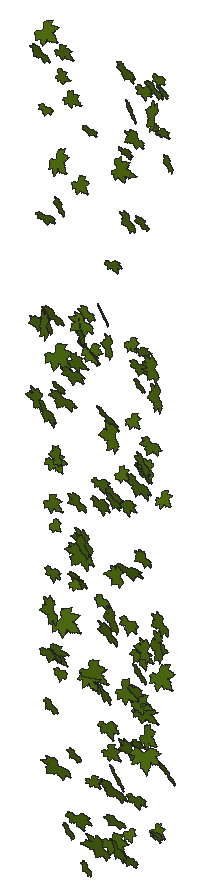
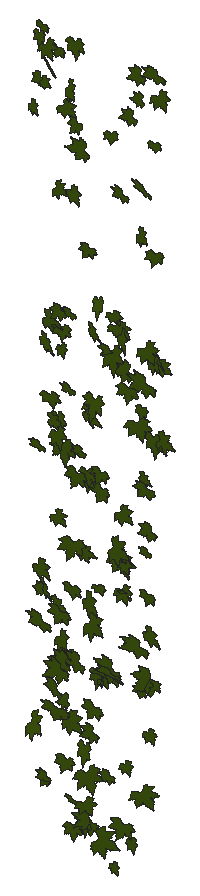
# SketchUp Ruby script. Lengths in inches.
U = 1.inch
M = Sketchup.active_model
def pt(a) = Geom::Point3d.new(a.map { |v| v * U })
def face(e, loops, mat)
  f = e.add_face(loops[0].map { |a| pt(a) })
  loops[1..].each { |l| e.add_face(l.map { |a| pt(a) }).erase! }
  f.material = f.back_material = mat if mat
  f
end
# faces: each face lists its corners as indices into pts; further lists are holes
def faces(e, pts, list, mat = nil) = list.each { |f| face(e, (f[0].is_a?(Array) ? f : [f]).map { |l| l.map { |i| pts[i] } }, mat) }
# xy, xz, yz: faces in a plane at the given z, y or x. An outline is a flat list of corners, or four numbers for a rectangle; further outlines are holes
def ring(l) = l.size == 4 ? [[l[0], l[1]], [l[2], l[1]], [l[2], l[3]], [l[0], l[3]]] : l.each_slice(2).to_a
def flat(e, list, mat, &to3) = list.each { |f| face(e, (f[0].is_a?(Array) ? f : [f]).map { |l| ring(l).map { |u, v| to3.(u, v) } }, mat) }
def xy(e, z, list, mat = nil) = flat(e, list, mat) { |x, y| [x, y, z] }
def xz(e, y, list, mat = nil) = flat(e, list, mat) { |x, z| [x, y, z] }
def yz(e, x, list, mat = nil) = flat(e, list, mat) { |y, z| [x, y, z] }
def lines(e, pts, list) = list.each { |a, b| e.add_line(pt(pts[a]), pt(pts[b])) }
# prism: a flat outline (further loops are holes) pulled along v
def prism(e, loops, v, mat = nil)
  f = face(e, loops, mat); d = Geom::Vector3d.new(v.map { |x| x * U })
  f.pushpull(f.normal.samedirection?(d) ? d.length : -d.length)
end
def box(e, o, s, mat = nil) = prism(e, [[o, [o[0] + s[0], o[1], o[2]], [o[0] + s[0], o[1] + s[1], o[2]], [o[0], o[1] + s[1], o[2]]]], [0, 0, s[2]], mat)
def at(x, y, z, deg = 0) = Geom::Transformation.translation(pt([x, y, z])) * Geom::Transformation.rotation(ORIGIN, Z_AXIS, deg.degrees)
def axes(o, x, y, z) = Geom::Transformation.new([*x, 0, *y, 0, *z, 0, *pt(o).to_a, 1])
def part(name) = M.definitions.add(name)
# library, detail: a bought-in or finely detailed component or shape, given as its bounding box
def library(name, o, s) = part(name).tap { |d| box(d.entities, o, s) }
def detail(e, o, s) = box(e.add_group.entities, o, s)
def put(e, d, t, mat = nil) = e.add_instance(d, t).tap { |i| i.material = mat if mat }
def group(e, t, mat = nil) = e.add_group.tap { |g| g.transformation = t; g.material = mat if mat }.entities
root = M.entities
M.materials.add("[Vegetation Blur 03]").color = [83, 114, 18]
c1 = part("ivy")
xy(c1.entities,0,[[0.782,0,0.786,0,0.787,0.005,0.789,0.009,0.821,0.072,0.875,0.147,1.001,0.272,1.073,0.331,1.137,0.363,1.178,0.379,1.223,0.384,1.272,0.383,1.311,0.374,1.36,0.355,1.399,0.334,1.491,0.285,1.541,0.244,1.583,0.199,1.617,0.15,1.64,0.128,1.662,0.115,1.717,0.105,1.745,0.093,1.784,0.054,1.819,0.057,1.854,0.064,1.882,0.075,1.896,0.074,1.91,0.071,1.937,0.063,1.964,0.053,1.99,0.038,2.016,0.015,2.034,0.002,2.04,0,2.038,0.003,2.036,0.007,2.033,0.038,2.036,0.068,2.045,0.1,2.055,0.116,2.064,0.123,2.077,0.129,2.088,0.129,2.106,0.132,2.118,0.13,2.179,0.132,2.207,0.133,2.225,0.133,2.242,0.138,2.22,0.162,2.207,0.186,2.206,0.213,2.212,0.236,2.228,0.262,2.247,0.274,2.298,0.283,2.355,0.294,2.37,0.296,2.376,0.295,2.377,0.3,2.377,0.303,2.385,0.329,2.411,0.37,2.426,0.392,2.449,0.407,2.511,0.426,2.561,0.444,2.619,0.466,2.589,0.469,2.561,0.476,2.501,0.5,2.449,0.516,2.424,0.523,2.401,0.535,2.377,0.556,2.372,0.568,2.36,0.575,2.268,0.586,2.225,0.592,2.207,0.599,2.194,0.61,2.143,0.65,2.13,0.664,2.122,0.682,2.123,0.7,2.13,0.719,2.148,0.75,2.17,0.781,2.195,0.807,2.221,0.828,2.284,0.874,2.291,0.88,2.288,0.887,2.276,0.9,2.267,0.916,2.265,0.933,2.273,0.967,2.292,1.002,2.313,1.03,2.334,1.054,2.348,1.067,2.358,1.074,2.363,1.076,2.362,1.081,2.35,1.094,2.347,1.11,2.35,1.143,2.359,1.18,2.385,1.254,2.415,1.324,2.448,1.393,2.45,1.4,2.446,1.398,2.44,1.394,2.427,1.383,2.402,1.36,2.376,1.339,2.345,1.324,2.305,1.309,2.282,1.303,2.273,1.306,2.245,1.294,2.212,1.287,2.187,1.291,2.163,1.301,2.142,1.316,2.134,1.327,2.124,1.325,2.09,1.292,2.053,1.259,2.014,1.234,1.973,1.215,1.954,1.21,1.931,1.208,1.909,1.212,1.893,1.22,1.879,1.233,1.872,1.248,1.867,1.281,1.864,1.319,1.821,1.258,1.773,1.197,1.726,1.141,1.698,1.121,1.679,1.116,1.666,1.117,1.647,1.122,1.632,1.129,1.62,1.141,1.617,1.154,1.617,1.219,1.621,1.254,1.623,1.268,1.623,1.281,1.618,1.314,1.606,1.346,1.603,1.375,1.607,1.403,1.603,1.467,1.599,1.499,1.605,1.525,1.614,1.552,1.629,1.577,1.635,1.589,1.629,1.587,1.618,1.582,1.596,1.566,1.581,1.556,1.568,1.552,1.557,1.55,1.545,1.553,1.531,1.562,1.522,1.572,1.504,1.591,1.486,1.611,1.474,1.631,1.457,1.666,1.455,1.684,1.457,1.698,1.452,1.715,1.444,1.728,1.424,1.754,1.419,1.772,1.423,1.786,1.434,1.819,1.444,1.848,1.446,1.855,1.44,1.861,1.43,1.867,1.386,1.904,1.349,1.948,1.326,1.973,1.31,1.995,1.288,2.048,1.284,2.153,1.287,2.254,1.284,2.255,1.282,2.253,1.278,2.247,1.274,2.237,1.266,2.216,1.226,2.125,1.208,2.076,1.184,2.033,1.155,1.984,1.135,1.942,1.111,1.899,1.083,1.861,1.053,1.85,1.059,1.83,1.061,1.809,1.056,1.79,1.049,1.767,1.04,1.749,1.018,1.733,0.994,1.726,0.942,1.734,0.95,1.6875,0.944,1.645,0.932,1.608,0.911,1.585,0.881,1.58,0.854,1.582,0.828,1.588,0.785,1.618,0.773,1.625,0.775,1.614,0.779,1.598,0.796,1.502,0.818,1.402,0.861,1.283,0.882,1.224,0.894,1.174,0.892,1.148,0.886,1.123,0.881,1.107,0.872,1.099,0.849,1.094,0.818,1.092,0.789,1.098,0.762,1.107,0.753,1.113,0.721,1.139,0.698,1.163,0.678,1.194,0.665,1.224,0.628,1.28,0.612,1.312,0.606,1.327,0.606,1.314,0.599,1.282,0.594,1.267,0.581,1.256,0.544,1.245,0.512,1.244,0.473,1.249,0.444,1.256,0.382,1.288,0.339,1.306,0.324,1.316,0.317,1.324,0.309,1.326,0.27,1.314,0.227,1.313,0.185,1.3125,0.152,1.317,0.122,1.328,0.092,1.345,0.073,1.353,0.079,1.338,0.092,1.308,0.117,1.249,0.13,1.215,0.139,1.164,0.147,1.148,0.157,1.136,0.163,1.122,0.174,1.086,0.177,1.067,0.182,1.054,0.186,1.043,0.191,1.038,0.211,1.028,0.237,1.005,0.25,0.974,0.253,0.96,0.25,0.944,0.242,0.914,0.243,0.906,0.249,0.902,0.26,0.894,0.289,0.88,0.307,0.873,0.322,0.862,0.364,0.799,0.403,0.738,0.431,0.709,0.439,0.691,0.441,0.678,0.4375,0.66,0.428,0.645,0.394,0.623,0.303,0.594,0.255,0.581,0.214,0.577,0.179,0.573,0.173,0.568,0.175,0.561,0.167,0.55,0.141,0.523,0.113,0.503,0.077,0.49,0.045,0.486,0.026,0.485,0.019,0.486,0.011,0.483,0,0.471,0.014,0.467,0.044,0.455,0.058,0.447,0.07,0.438,0.097,0.411,0.125,0.394,0.158,0.377,0.174,0.366,0.182,0.359,0.185,0.361,0.242,0.331,0.253,0.316,0.258,0.303,0.262,0.283,0.274,0.278,0.308,0.274,0.341,0.252,0.366,0.226,0.366,0.222,0.37,0.22,0.38,0.221,0.395,0.221,0.425,0.216,0.45,0.207,0.465,0.192,0.473,0.178,0.484,0.15,0.489,0.116,0.483,0.089,0.468,0.058,0.45,0.035,0.435,0.018,0.429,0.011,0.434,0.012,0.438,0.014,0.469,0.019,0.542,0.016,0.581,0.015,0.612,0.027,0.68,0.055,0.696,0.057,0.712,0.052,0.73,0.045,0.741,0.036,0.766,0.014]])
put(root,c1,axes([11.16,173.7,30.11],[0.07342,0.0201,-0.45241],[-0.55143,0.12193,-0.05876],[-0.05747,-1.14418,-0.01421]),"[Vegetation Blur 03]")
put(root,c1,axes([11,173.7,33.93],[0.13601,0.05917,-0.30855],[-0.37908,0.03752,-0.11017],[-0.00748,-0.82593,-0.02711]),"[Vegetation Blur 03]")
put(root,c1,axes([10.83,173.7,48.26],[0.33145,0.05992,-0.29685],[-0.36343,0.14447,-0.2657],[-0.03257,-1.00226,-0.05605]),"[Vegetation Blur 03]")
put(root,c1,axes([11.58,173.7,34.26],[0.12192,-0.00071,-0.41999],[-0.49465,0.29998,-0.09572],[-0.14193,-1.04612,-0.02717]),"[Vegetation Blur 03]")
put(root,c1,axes([11.62,173.7,34.28],[0.14174,-0.20689,-0.42841],[-0.51411,0.25268,-0.13249],[-0.14609,-1.08996,0.0506]),"[Vegetation Blur 03]")
put(root,c1,axes([10.85,173.7,39.43],[0.38883,0.03177,-0.00541],[-0.00902,0.12865,-0.31342],[0.01417,-0.78985,-0.05127]),"[Vegetation Blur 03]")
put(root,c1,axes([11.09,173.7,45.22],[0.29737,0.00668,-0.03254],[-0.03987,-0.00069,-0.24271],[0.00326,-0.6174,-0.00008]),"[Vegetation Blur 03]")
put(root,c1,axes([10.63,173.7,48.53],[0.22945,0.18892,0.3925],[0.48869,-0.02142,-0.18866],[0.02999,-1.09631,0.07132]),"[Vegetation Blur 03]")
put(root,c1,axes([11.57,173.7,34.72],[0.32489,0.11128,-0.34401],[-0.42351,0.17483,-0.25752],[-0.03505,-1.08109,-0.07706]),"[Vegetation Blur 03]")
put(root,c1,axes([11.04,173.7,29.73],[0.57169,-0.21875,-0.18427],[-0.21197,0.1873,-0.473],[-0.13171,-1.2509,-0.0386]),"[Vegetation Blur 03]")
put(root,c1,axes([11.55,173.7,14.08],[0.26898,-0.00531,-0.22272],[-0.27011,0.10743,-0.21769],[-0.03898,-0.78115,-0.02842]),"[Vegetation Blur 03]")
put(root,c1,axes([11.86,173.7,19.51],[0.26861,-0.16753,-0.42435],[-0.51691,0.14174,-0.22674],[-0.09889,-1.19591,0.03257]),"[Vegetation Blur 03]")
put(root,c1,axes([11.67,173.7,11.125],[0.44397,0.1395,-0.34863],[-0.43136,0.05055,-0.3627],[0.03168,-1.26682,-0.05286]),"[Vegetation Blur 03]")
put(root,c1,axes([11.64,173.7,16.72],[0.30297,0.01543,-0.16149],[-0.19571,0.1367,-0.2425],[-0.03016,-0.73198,-0.04869]),"[Vegetation Blur 03]")
put(root,c1,axes([12.27,173.7,40.52],[0.10541,0.02404,-0.33372],[-0.3979,0.2077,-0.08136],[-0.09494,-0.84377,-0.02954]),"[Vegetation Blur 03]")
put(root,c1,axes([11.22,173.7,24.11],[0.22933,0.01454,0.32661],[0.40022,0.004,-0.18721],[0.0052,-0.94915,0.00421]),"[Vegetation Blur 03]")
put(root,c1,axes([11.4,173.7,21.01],[0.4011,-0.07198,0.04538],[0.05521,-0.01426,-0.32859],[-0.0356,-0.83315,0.0017]),"[Vegetation Blur 03]")
put(root,c1,axes([10.88,173.7,16.34],[0.50593,-0.03643,0.3437],[0.41936,0.17969,-0.40818],[0.0424,-1.34262,-0.06395]),"[Vegetation Blur 03]")
put(root,c1,axes([12.28,173.7,27.52],[0.12968,-0.11784,-0.31424],[-0.38451,0.09135,-0.11108],[-0.06065,-0.83104,0.03235]),"[Vegetation Blur 03]")
put(root,c1,axes([11.58,173.7,23.08],[0.14273,0.06127,0.20808],[0.25666,-0.04237,-0.11531],[-0.00355,-0.59977,0.0294]),"[Vegetation Blur 03]")
put(root,c1,axes([11.28,173.7,26.49],[0.3729,0.07352,0.23123],[0.28448,-0.01242,-0.30497],[0.02479,-0.96364,0.02157]),"[Vegetation Blur 03]")
put(root,c1,axes([11.84,173.7,30.48],[0.49872,0.09657,-0.2358],[-0.29251,0.12066,-0.4043],[0.0109,-1.17989,-0.06065]),"[Vegetation Blur 03]")
put(root,c1,axes([11.83,173.7,30.86],[0.33145,-0.08577,-0.02014],[-0.01771,0.11215,-0.26935],[-0.04508,-0.6747,-0.04221]),"[Vegetation Blur 03]")
put(root,c1,axes([11.1875,173.7,31.82],[0.38163,0.10723,0.44815],[0.5511,-0.01709,-0.31195],[0.0229,-1.37595,0.0388]),"[Vegetation Blur 03]")
put(root,c1,axes([11.51,173.7,42.07],[0.21319,0.1755,0.40106],[0.49372,-0.23014,-0.15897],[-0.07069,-1.078,0.09923]),"[Vegetation Blur 03]")
put(root,c1,axes([11.95,173.7,15.84],[0.32221,-0.0387,0.02273],[0.02664,-0.04287,-0.26295],[-0.0205,-0.66413,0.01565]),"[Vegetation Blur 03]")
put(root,c1,axes([12.03,173.7,46.77],[0.07701,-0.01607,0.28736],[0.35217,-0.0014,-0.06288],[-0.00233,-0.74167,-0.00611]),"[Vegetation Blur 03]")
put(root,c1,axes([11.58,173.7,17.75],[0.25598,0.2014,0.48378],[0.59803,0.04143,-0.21349],[0.05748,-1.32803,0.06671]),"[Vegetation Blur 03]")
put(root,c1,axes([11.89,173.7,48.13],[0.23882,-0.04134,0.29544],[0.36225,0.06442,-0.19363],[0.01513,-0.89011,-0.02773]),"[Vegetation Blur 03]")
put(root,c1,axes([12.58,173.7,7.89],[0.29522,-0.08617,-0.18688],[-0.21829,0.16177,-0.24143],[-0.08083,-0.75161,-0.03054]),"[Vegetation Blur 03]")
put(root,c1,axes([12.34,173.7,31.86],[0.50551,0.02715,-0.04471],[-0.05585,0.1053,-0.41049],[0.00753,-1.04102,-0.04269]),"[Vegetation Blur 03]")
put(root,c1,axes([12.92,173.7,11.91],[0.2455,0.02361,-0.20397],[-0.24867,0.10235,-0.19749],[-0.02754,-0.71362,-0.03507]),"[Vegetation Blur 03]")
put(root,c1,axes([12.96,173.7,22.6],[0.23892,0.03876,-0.2007],[-0.24369,0.14566,-0.1888],[-0.038,-0.69034,-0.0511]),"[Vegetation Blur 03]")
put(root,c1,axes([13.23,173.7,25.42],[0.22065,0.07279,-0.34055],[-0.41864,0.06201,-0.17859],[-0.01021,-0.96933,-0.037]),"[Vegetation Blur 03]")
put(root,c1,axes([12.4,173.7,45.74],[0.16739,0.00231,0.3142],[0.38437,0.04772,-0.13645],[0.02172,-0.86254,-0.00671]),"[Vegetation Blur 03]")
put(root,c1,axes([12.97,173.7,21.24],[0.33471,0.047,-0.24757],[-0.30145,0.17573,-0.26622],[-0.0408,-0.91277,-0.064]),"[Vegetation Blur 03]")
put(root,c1,axes([12.74,173.7,20.37],[0.12441,0.10653,0.22366],[0.27873,-0.02631,-0.1013],[0.00957,-0.61876,0.04281]),"[Vegetation Blur 03]")
put(root,c1,axes([13.86,173.7,23.6],[0.10808,0.0782,-0.51354],[-0.62715,0.14615,-0.08441],[-0.06373,-1.30565,-0.04021]),"[Vegetation Blur 03]")
put(root,c1,axes([12.96,173.7,22.875],[0.56655,-0.0115,-0.27779],[-0.34007,0.04247,-0.46224],[-0.01542,-1.35941,-0.01209]),"[Vegetation Blur 03]")
put(root,c1,axes([13.29,173.7,34.89],[0.41729,-0.27977,-0.39423],[-0.44817,0.37379,-0.3577],[-0.22574,-1.25924,-0.01859]),"[Vegetation Blur 03]")
put(root,c1,axes([12.51,173.7,8.41],[0.53014,0.02962,0.10212],[0.12282,0.12551,-0.4304],[0.02794,-1.11386,-0.04578]),"[Vegetation Blur 03]")
put(root,c1,axes([13.65,173.7,23.35],[0.21226,-0.08156,-0.39258],[-0.47103,0.20087,-0.17619],[-0.10528,-1.06312,-0.00317]),"[Vegetation Blur 03]")
put(root,c1,axes([12.71,173.7,31.98],[0.16066,-0.07376,0.37357],[0.45903,0.04715,-0.13002],[0.00982,-0.99714,-0.03378]),"[Vegetation Blur 03]")
put(root,c1,axes([13.39,173.7,35.1],[0.38856,-0.00058,-0.29483],[-0.35992,-0.09405,-0.31593],[0.03091,-1.0877,0.02748]),"[Vegetation Blur 03]")
put(root,c1,axes([12.87,173.7,41.5],[0.24024,0.06291,0.29442],[0.3619,-0.06648,-0.19446],[-0.01006,-0.88941,0.03536]),"[Vegetation Blur 03]")
put(root,c1,axes([13.41,173.7,33.74],[0.55985,-0.09656,-0.30764],[-0.35518,0.35678,-0.44814],[-0.13469,-1.34226,-0.09699]),"[Vegetation Blur 03]")
put(root,c1,axes([13.73,173.7,6.25],[0.22842,-0.06235,-0.19773],[-0.23665,0.11144,-0.18763],[-0.06007,-0.67607,-0.01269]),"[Vegetation Blur 03]")
put(root,c1,axes([13.64,173.7,35.52],[0.31144,-0.00755,-0.1936],[-0.23722,0.00118,-0.25419],[-0.00327,-0.80561,0.00144]),"[Vegetation Blur 03]")
put(root,c1,axes([13.61,173.7,44.96],[0.30877,0.02964,-0.06253],[-0.07793,0.09874,-0.24894],[0.00225,-0.64717,-0.04084]),"[Vegetation Blur 03]")
put(root,c1,axes([14.74,173.7,7.86],[0.10967,0.16764,-0.53959],[-0.66571,-0.0227,-0.09123],[0.02429,-1.37893,-0.0641]),"[Vegetation Blur 03]")
put(root,c1,axes([13.22,173.7,15.87],[0.43423,0.11965,0.28912],[0.35873,-0.10053,-0.35232],[0.01383,-1.14881,0.06094]),"[Vegetation Blur 03]")
put(root,c1,axes([13.45,173.7,32.98],[0.34318,0.09184,0.26358],[0.326,-0.10859,-0.27677],[-0.00403,-0.96364,0.05631]),"[Vegetation Blur 03]")
put(root,c1,axes([13.7,173.7,10.47],[0.24944,0.02336,0.19362],[0.23616,0.05082,-0.20362],[0.02524,-0.70655,-0.00824]),"[Vegetation Blur 03]")
put(root,c1,axes([14.39,173.7,15.9],[0.17883,0.01791,-0.19414],[-0.23754,0.05276,-0.14498],[-0.01529,-0.61012,-0.01823]),"[Vegetation Blur 03]")
put(root,c1,axes([13.29,173.7,15.91],[0.34678,0.03788,0.46084],[0.56412,0.05104,-0.28341],[0.03077,-1.36263,0.00219]),"[Vegetation Blur 03]")
put(root,c1,axes([15.08,173.7,19.15],[0.17288,0.13727,-0.46997],[-0.57483,0.20036,-0.13164],[-0.0749,-1.22089,-0.07445]),"[Vegetation Blur 03]")
put(root,c1,axes([14.09,173.7,26.55],[0.40772,-0.01716,0.08723],[0.10718,0.04684,-0.33224],[-0.00228,-0.8661,-0.01969]),"[Vegetation Blur 03]")
put(root,c1,axes([14.53,173.7,20.62],[0.28445,-0.01133,-0.1134],[-0.139,-0.04223,-0.23156],[0.00407,-0.65007,0.01702]),"[Vegetation Blur 03]")
put(root,c1,axes([14.47,173.7,35.88],[0.40706,-0.21039,-0.21028],[-0.21941,0.3311,-0.33502],[-0.1694,-0.93442,-0.07136]),"[Vegetation Blur 03]")
put(root,c1,axes([14.06,173.7,25.625],[0.48848,-0.12647,0.08295],[0.10536,0.05262,-0.40062],[-0.05484,-1.02537,-0.03079]),"[Vegetation Blur 03]")
put(root,c1,axes([14.47,173.7,15.94],[0.464,-0.18688,-0.09777],[-0.10719,0.14954,-0.38378],[-0.10541,-0.97473,-0.04013]),"[Vegetation Blur 03]")
put(root,c1,axes([15.33,173.7,34.38],[0.12813,-0.15006,-0.36786],[-0.44192,0.20151,-0.11546],[-0.11482,-0.94298,0.03387]),"[Vegetation Blur 03]")
put(root,c1,axes([14.77,173.7,11.03],[0.53027,0.09687,-0.32245],[-0.39653,0.24084,-0.42296],[-0.03295,-1.33931,-0.09938]),"[Vegetation Blur 03]")
put(root,c1,axes([14.39,173.7,30.54],[0.61753,-0.18671,-0.12394],[-0.12621,0.33022,-0.49708],[-0.12397,-1.26626,-0.11135]),"[Vegetation Blur 03]")
put(root,c1,axes([15.35,173.7,20.17],[0.24952,-0.09563,-0.45788],[-0.54485,0.27669,-0.20686],[-0.14163,-1.23287,-0.01091]),"[Vegetation Blur 03]")
put(root,c1,axes([15.14,173.7,9.23],[0.30579,0.15468,-0.23311],[-0.2938,0.07258,-0.24913],[0.03027,-0.858,-0.0631]),"[Vegetation Blur 03]")
put(root,c1,axes([15.6,173.7,29.98],[0.21628,-0.19716,-0.4852],[-0.59473,0.13393,-0.18514],[-0.09444,-1.29492,0.05473]),"[Vegetation Blur 03]")
put(root,c1,axes([14.42,173.7,13.84],[0.46672,-0.03992,0.15461],[0.18977,0.01161,-0.3811],[-0.01585,-1.03645,-0.01022]),"[Vegetation Blur 03]")
put(root,c1,axes([14.8,173.7,38.17],[0.33638,0.01493,0.11781],[0.14294,0.07701,-0.27338],[0.02139,-0.74929,-0.02575]),"[Vegetation Blur 03]")
put(root,c1,axes([14.66,173.7,12.24],[0.25126,-0.00237,0.3092],[0.37875,0.02524,-0.20497],[0.00958,-0.93516,-0.00632]),"[Vegetation Blur 03]")
put(root,c1,axes([15.02,173.7,26.54],[0.44154,-0.10792,-0.13293],[-0.15664,0.11844,-0.36167],[-0.06888,-0.96117,-0.02964]),"[Vegetation Blur 03]")
put(root,c1,axes([15.04,173.7,26.13],[0.39751,-0.09835,-0.09675],[-0.112,0.11608,-0.32505],[-0.0616,-0.84567,-0.03337]),"[Vegetation Blur 03]")
put(root,c1,axes([15.92,173.7,22.44],[0.06394,-0.03491,-0.38067],[-0.46672,-0.01334,-0.05203],[0.00412,-0.96871,0.01444]),"[Vegetation Blur 03]")
put(root,c1,axes([14.5625,173.7,7.51],[0.43162,0.02667,0.37239],[0.45622,0.01814,-0.35241],[0.01531,-1.29236,0.00274]),"[Vegetation Blur 03]")
put(root,c1,axes([15.21,173.7,11.9],[0.51252,-0.27009,-0.18144],[-0.18784,0.30748,-0.42542],[-0.17711,-1.10772,-0.07385]),"[Vegetation Blur 03]")
put(root,c1,axes([15.28,173.7,8.04],[0.4822,-0.17189,-0.16775],[-0.19534,0.15084,-0.39833],[-0.10519,-1.06807,-0.02926]),"[Vegetation Blur 03]")
put(root,c1,axes([15.43,173.7,27.02],[0.11399,0.08931,0.26369],[0.32563,0.00233,-0.09389],[0.01551,-0.70503,0.03309]),"[Vegetation Blur 03]")
put(root,c1,axes([16.25,173.7,13.51],[0.24902,0.09318,-0.40988],[-0.50306,0.12516,-0.1991],[-0.03467,-1.14673,-0.05504]),"[Vegetation Blur 03]")
put(root,c1,axes([15.26,173.7,42.76],[0.09049,0.02962,0.47011],[0.57571,0.04471,-0.07426],[0.0237,-1.19903,0.00884]),"[Vegetation Blur 03]")
put(root,c1,axes([16.375,173.7,46.97],[0.14161,0.02749,-0.37414],[-0.43235,0.33737,-0.1051],[-0.153,-0.92792,-0.0493]),"[Vegetation Blur 03]")
put(root,c1,axes([15.64,173.7,49.125],[0.51011,-0.11701,-0.13612],[-0.15838,0.15628,-0.41647],[-0.07724,-1.09327,-0.04497]),"[Vegetation Blur 03]")
put(root,c1,axes([16.14,173.7,41.34],[0.31562,-0.0779,-0.30416],[-0.3657,0.1532,-0.25894],[-0.08116,-0.99323,-0.01608]),"[Vegetation Blur 03]")
put(root,c1,axes([15.75,173.7,7.54],[0.43132,0.00683,-0.12215],[-0.14822,0.15148,-0.34728],[-0.02104,-0.9272,-0.05763]),"[Vegetation Blur 03]")
put(root,c1,axes([15.4375,173.7,22.54],[0.54712,0.06533,0.00829],[0.00324,0.23778,-0.43729],[0.03318,-1.10066,-0.09398]),"[Vegetation Blur 03]")
put(root,c1,axes([15.39,173.7,26.03],[0.51598,-0.04836,0.08245],[0.10256,0.07999,-0.4201],[-0.01553,-1.07898,-0.03484]),"[Vegetation Blur 03]")
put(root,c1,axes([15.63,173.7,44.5],[0.35213,-0.1038,0.09821],[0.12718,0.11373,-0.28482],[-0.02917,-0.75727,-0.05624]),"[Vegetation Blur 03]")
put(root,c1,axes([15.47,173.7,15.54],[0.19537,0.05525,0.44525],[0.54604,-0.05051,-0.1586],[-0.01409,-1.19141,0.02737]),"[Vegetation Blur 03]")
put(root,c1,axes([15.85,173.7,19.97],[0.45876,-0.06676,-0.02085],[-0.02631,-0.02088,-0.37522],[-0.03182,-0.94526,0.00976]),"[Vegetation Blur 03]")
put(root,c1,axes([15.95,173.7,8.47],[0.21181,0.06558,0.16158],[0.19963,-0.12494,-0.16633],[-0.01894,-0.58339,0.05378]),"[Vegetation Blur 03]")
put(root,c1,axes([16.59,173.7,45.78],[0.26725,0.04128,-0.32232],[-0.39537,0.00799,-0.21819],[0.00802,-0.98126,-0.01534]),"[Vegetation Blur 03]")
put(root,c1,axes([15.99,173.7,34.23],[0.21448,0.07418,0.20841],[0.25788,-0.06923,-0.1729],[-0.00284,-0.68276,0.04017]),"[Vegetation Blur 03]")
put(root,c1,axes([16.8125,173.7,17.58],[0.21131,0.04206,-0.34485],[-0.41038,0.25638,-0.16258],[-0.10272,-0.93777,-0.05992]),"[Vegetation Blur 03]")
put(root,c1,axes([16.05,173.7,30.15],[0.18344,0.08958,0.24161],[0.29922,-0.05038,-0.14838],[0.0019,-0.7149,0.04073]),"[Vegetation Blur 03]")
put(root,c1,axes([16.13,173.7,10.68],[0.44484,-0.01751,0.04002],[0.04967,0.10203,-0.36079],[-0.00297,-0.91526,-0.04099]),"[Vegetation Blur 03]")
put(root,c1,axes([16.19,173.7,16.36],[0.36338,-0.06137,0.0857],[0.10665,0.03955,-0.29676],[-0.02326,-0.77736,-0.02186]),"[Vegetation Blur 03]")
put(root,c1,axes([16.23,173.7,27.66],[0.62172,-0.07982,-0.18766],[-0.22411,0.16779,-0.50577],[-0.06444,-1.35373,-0.05162]),"[Vegetation Blur 03]")
put(root,c1,axes([16.73,173.7,32.71],[0.25042,-0.03463,-0.18206],[-0.21423,0.16131,-0.2011],[-0.06442,-0.671,-0.03895]),"[Vegetation Blur 03]")
put(root,c1,axes([17.17,173.7,41.26],[0.07231,0.11382,-0.30015],[-0.37128,0.06711,-0.05557],[-0.02172,-0.76837,-0.04931]),"[Vegetation Blur 03]")
put(root,c1,axes([16.4,173.7,33.65],[0.43667,-0.00599,-0.05285],[-0.0643,0.07555,-0.35518],[-0.00825,-0.90526,-0.02929]),"[Vegetation Blur 03]")
put(root,c1,axes([16.8125,173.7,28.3],[0.37381,-0.01776,-0.27785],[-0.3272,0.26974,-0.29592],[-0.09444,-1.00486,-0.07453]),"[Vegetation Blur 03]")
put(root,c1,axes([16.51,173.7,13.36],[0.12453,-0.12682,0.21988],[0.27637,0.0612,-0.0987],[0.00185,-0.60769,-0.05583]),"[Vegetation Blur 03]")
put(root,c1,axes([17.08,173.7,23.83],[0.24891,0.01709,-0.28911],[-0.35411,0.04401,-0.20266],[-0.01273,-0.88984,-0.01558]),"[Vegetation Blur 03]")
put(root,c1,axes([17.53,173.7,19.13],[0.07751,-0.08641,-0.39879],[-0.48715,0.10409,-0.06661],[-0.05668,-1.01274,0.02718]),"[Vegetation Blur 03]")
put(root,c1,axes([16.88,173.7,28.97],[0.45681,-0.21004,-0.23078],[-0.27305,0.15298,-0.3819],[-0.12578,-1.09491,-0.00909]),"[Vegetation Blur 03]")
put(root,c1,axes([16.44,173.7,15.1875],[0.0827,0.01826,0.45445],[0.55686,-0.01784,-0.06738],[-0.00727,-1.15829,0.0082]),"[Vegetation Blur 03]")
put(root,c1,axes([16.33,173.7,18.28],[0.50405,-0.0121,0.1413],[0.17315,0.00073,-0.4114],[-0.00545,-1.09673,-0.00183]),"[Vegetation Blur 03]")
put(root,c1,axes([16.57,173.7,34.17],[0.30561,-0.04373,0.17256],[0.21196,0.11676,-0.24539],[0.01507,-0.75575,-0.0479]),"[Vegetation Blur 03]")
put(root,c1,axes([16.72,173.7,48.17],[0.38022,-0.03036,0.06928],[0.08439,-0.02832,-0.31043],[-0.01739,-0.80118,0.00835]),"[Vegetation Blur 03]")
put(root,c1,axes([17.75,173.7,28.72],[0.06632,-0.08264,-0.34848],[-0.42857,0.02082,-0.0551],[-0.0162,-0.88896,0.0311]),"[Vegetation Blur 03]")
put(root,c1,axes([16.35,173.7,14.95],[0.37722,-0.01424,0.37521],[0.45787,0.12358,-0.30587],[0.04206,-1.2175,-0.03543]),"[Vegetation Blur 03]")
put(root,c1,axes([16.375,173.7,13.12],[0.61342,0.08443,0.16311],[0.20359,-0.16924,-0.49623],[0.01316,-1.31678,0.07424]),"[Vegetation Blur 03]")
put(root,c1,axes([17.9,173.7,34.22],[0.15478,-0.07462,-0.45486],[-0.55676,0.07347,-0.12809],[-0.04416,-1.18802,0.02065]),"[Vegetation Blur 03]")
put(root,c1,axes([17.51,173.7,48.67],[0.32569,0.04627,-0.29452],[-0.35796,0.18221,-0.25916],[-0.05099,-0.98359,-0.06186]),"[Vegetation Blur 03]")
put(root,c1,axes([17.16,173.7,29.87],[0.44969,-0.01244,-0.10758],[-0.13185,-0.00591,-0.36702],[-0.00499,-0.96429,0.00364]),"[Vegetation Blur 03]")
put(root,c1,axes([18.1,173.7,47.54],[0.07293,-0.28065,-0.423],[-0.50755,0.30955,-0.09059],[-0.17213,-1.03162,0.0879]),"[Vegetation Blur 03]")
put(root,c1,axes([16.9,173.7,13.63],[0.13579,0.06981,0.42324],[0.51409,-0.17958,-0.1052],[-0.07611,-1.08841,0.0445]),"[Vegetation Blur 03]")
put(root,c1,axes([17.98,173.7,46.51],[0.10604,0.023,-0.23018],[-0.28135,0.05824,-0.08542],[-0.02259,-0.61729,-0.01663]),"[Vegetation Blur 03]")
put(root,c1,axes([18.08,173.7,32.93],[0.29092,-0.24551,-0.40873],[-0.49509,0.19114,-0.25278],[-0.14116,-1.1764,0.04423]),"[Vegetation Blur 03]")
put(root,c1,axes([18.24,173.7,19.91],[0.26701,-0.30376,-0.4486],[-0.53833,0.27065,-0.24226],[-0.1847,-1.22801,0.05757]),"[Vegetation Blur 03]")
put(root,c1,axes([18.5,173.7,12.76],[0.09506,0.21771,-0.46057],[-0.55663,0.32363,-0.05246],[-0.14082,-1.13231,-0.10355]),"[Vegetation Blur 03]")
put(root,c1,axes([18.13,173.7,20.89],[0.30205,-0.06223,-0.36549],[-0.44449,0.11303,-0.2477],[-0.06243,-1.1058,-0.00475]),"[Vegetation Blur 03]")
put(root,c1,axes([17.56,173.7,9.14],[0.28399,-0.06546,0.07539],[0.09562,0.06624,-0.23087],[-0.02006,-0.61097,-0.03311]),"[Vegetation Blur 03]")
put(root,c1,axes([17.49,173.7,9.02],[0.18546,0.05213,0.26962],[0.33131,-0.03649,-0.15069],[-0.00311,-0.77875,0.02511]),"[Vegetation Blur 03]")
put(root,c1,axes([17.71,173.7,49.09],[0.3174,-0.05029,0.04385],[0.05287,-0.02687,-0.25971],[-0.02626,-0.66189,0.00721]),"[Vegetation Blur 03]")
put(root,c1,axes([17.95,173.7,48.76],[0.35771,-0.12648,-0.10441],[-0.11497,0.1604,-0.29291],[-0.08323,-0.76513,-0.04414]),"[Vegetation Blur 03]")
put(root,c1,axes([17.8,173.7,26.53],[0.15249,0.14355,0.27563],[0.34484,-0.05498,-0.12257],[0.00385,-0.76056,0.06089]),"[Vegetation Blur 03]")
put(root,c1,axes([17.39,173.7,17.11],[0.33086,0.13392,0.42114],[0.51995,-0.11554,-0.26631],[-0.01255,-1.25609,0.0694]),"[Vegetation Blur 03]")
put(root,c1,axes([17.91,173.7,46.08],[0.20167,-0.04503,0.17751],[0.21848,0.0617,-0.16287],[0.00725,-0.60725,-0.02971]),"[Vegetation Blur 03]")
put(root,c1,axes([18.04,173.7,18.78],[0.04043,-0.04833,0.23762],[0.29161,-0.02839,-0.03396],[-0.01694,-0.60422,-0.01741]),"[Vegetation Blur 03]")
put(root,c1,axes([18.63,173.7,45.07],[0.17412,-0.05091,-0.27988],[-0.33267,0.17495,-0.14285],[-0.08689,-0.77186,-0.01392]),"[Vegetation Blur 03]")
